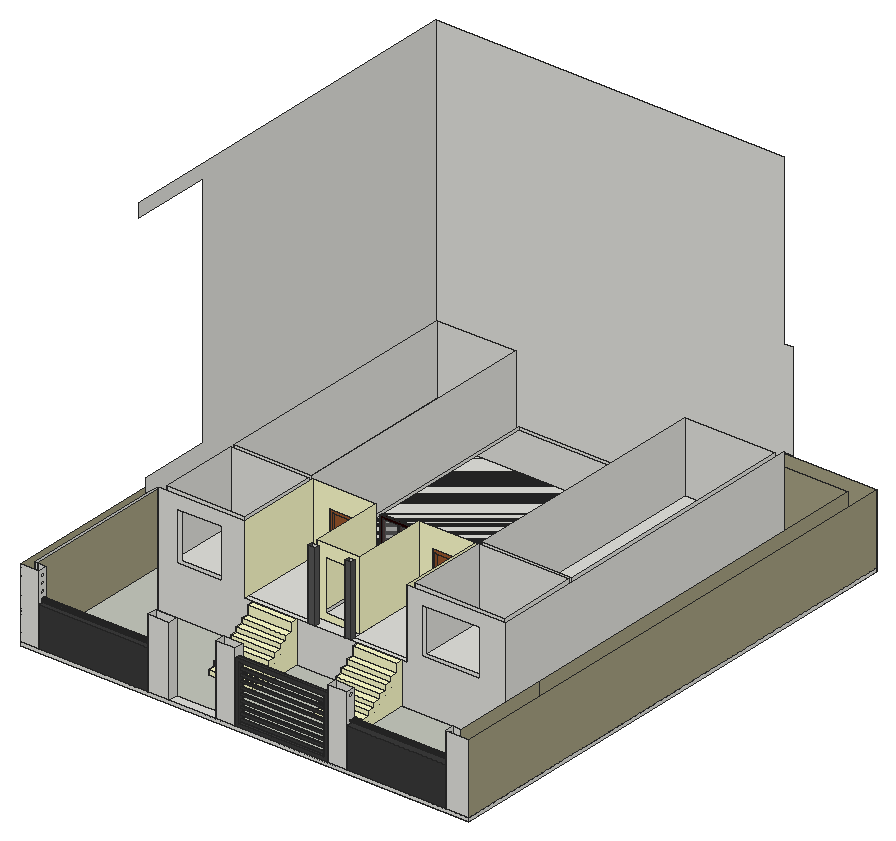
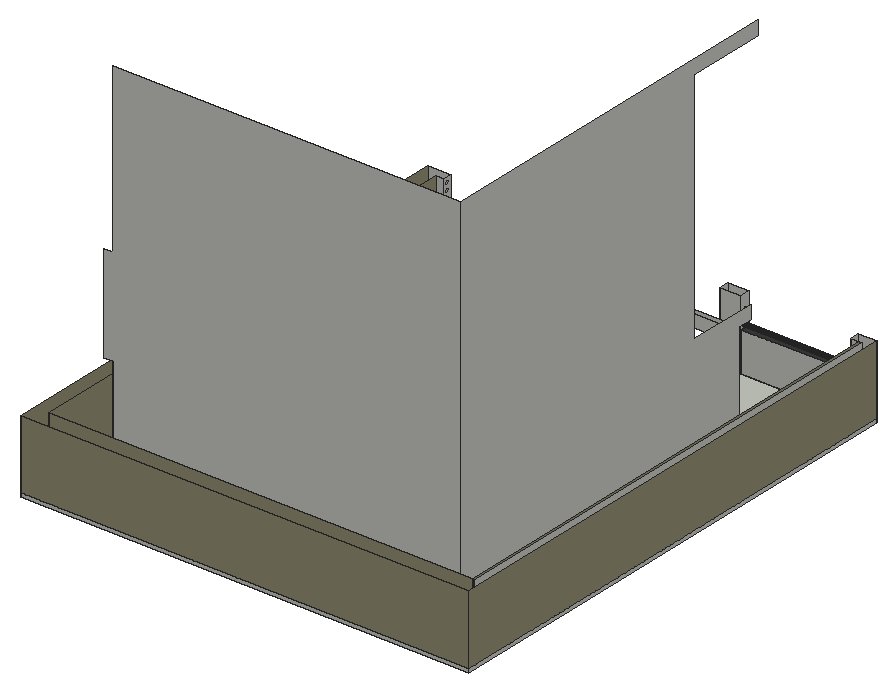
# SketchUp Ruby script. Lengths in inches.
U = 1.inch
M = Sketchup.active_model
def pt(a) = Geom::Point3d.new(a.map { |v| v * U })
def face(e, loops, mat)
  f = e.add_face(loops[0].map { |a| pt(a) })
  loops[1..].each { |l| e.add_face(l.map { |a| pt(a) }).erase! }
  f.material = f.back_material = mat if mat
  f
end
# faces: each face lists its corners as indices into pts; further lists are holes
def faces(e, pts, list, mat = nil) = list.each { |f| face(e, (f[0].is_a?(Array) ? f : [f]).map { |l| l.map { |i| pts[i] } }, mat) }
# xy, xz, yz: faces in a plane at the given z, y or x. An outline is a flat list of corners, or four numbers for a rectangle; further outlines are holes
def ring(l) = l.size == 4 ? [[l[0], l[1]], [l[2], l[1]], [l[2], l[3]], [l[0], l[3]]] : l.each_slice(2).to_a
def flat(e, list, mat, &to3) = list.each { |f| face(e, (f[0].is_a?(Array) ? f : [f]).map { |l| ring(l).map { |u, v| to3.(u, v) } }, mat) }
def xy(e, z, list, mat = nil) = flat(e, list, mat) { |x, y| [x, y, z] }
def xz(e, y, list, mat = nil) = flat(e, list, mat) { |x, z| [x, y, z] }
def yz(e, x, list, mat = nil) = flat(e, list, mat) { |y, z| [x, y, z] }
def lines(e, pts, list) = list.each { |a, b| e.add_line(pt(pts[a]), pt(pts[b])) }
# prism: a flat outline (further loops are holes) pulled along v
def prism(e, loops, v, mat = nil)
  f = face(e, loops, mat); d = Geom::Vector3d.new(v.map { |x| x * U })
  f.pushpull(f.normal.samedirection?(d) ? d.length : -d.length)
end
def box(e, o, s, mat = nil) = prism(e, [[o, [o[0] + s[0], o[1], o[2]], [o[0] + s[0], o[1] + s[1], o[2]], [o[0], o[1] + s[1], o[2]]]], [0, 0, s[2]], mat)
def at(x, y, z, deg = 0) = Geom::Transformation.translation(pt([x, y, z])) * Geom::Transformation.rotation(ORIGIN, Z_AXIS, deg.degrees)
def axes(o, x, y, z) = Geom::Transformation.new([*x, 0, *y, 0, *z, 0, *pt(o).to_a, 1])
def part(name) = M.definitions.add(name)
# library, detail: a bought-in or finely detailed component or shape, given as its bounding box
def library(name, o, s) = part(name).tap { |d| box(d.entities, o, s) }
def detail(e, o, s) = box(e.add_group.entities, o, s)
def put(e, d, t, mat = nil) = e.add_instance(d, t).tap { |i| i.material = mat if mat }
def group(e, t, mat = nil) = e.add_group.tap { |g| g.transformation = t; g.material = mat if mat }.entities
root = M.entities
M.materials.add("[Color A08]").color = [30, 0, 0]
M.materials.add("[Color E01]").color = [255, 255, 204]
M.materials.add("[Color M06]").color = [86, 86, 86]
M.materials.add("[Color M07]").color = [58, 58, 58]
M.materials.add("[Pavers with Grass Herringbone]").color = [197, 201, 190]
M.materials.add("[Stone Coursed Rough]").color = [165, 160, 130]
M.materials.add("[Translucent Glass Gray]").color = [128, 128, 128]
M.materials["[Translucent Glass Gray]"].alpha = 0.5
M.materials.add("[Wood Cherry Original]").color = [152, 86, 42]
c1 = part("Group\#3")
xy(c1.entities,0,[[0,0,60.375,4]])
xy(c1.entities,4.67,[[4.67,0,28.45,4],[32.75,0,55.71,4]],"[Color A08]")
xy(c1.entities,93.02,[[4.67,0,28.45,4],[32.75,0,55.71,4]])
xy(c1.entities,97.6875,[[0,0,60.375,4]],"[Color A08]")
xz(c1.entities,0,[[[0,0,60.375,97.6875],[4.67,4.67,28.45,93.02],[32.75,4.67,55.71,93.02]]],"[Color A08]")
xz(c1.entities,0,[[4.67,4.67,28.45,93.02],[32.75,4.67,55.71,93.02]],"[Translucent Glass Gray]")
xz(c1.entities,4,[[[0,0,60.375,97.6875],[4.67,4.67,28.45,93.02],[32.75,4.67,55.71,93.02]]],"[Color A08]")
yz(c1.entities,0,[[0,0,4,97.6875]],"[Color A08]")
yz(c1.entities,4.67,[[0,4.67,4,93.02]],"[Color A08]")
yz(c1.entities,28.45,[[0,4.67,4,93.02]],"[Color A08]")
yz(c1.entities,32.75,[[0,4.67,4,93.02]],"[Color A08]")
yz(c1.entities,55.71,[[0,4.67,4,93.02]],"[Color A08]")
yz(c1.entities,60.375,[[0,0,4,97.6875]],"[Color A08]")
c2 = part("Group\#1")
xy(c2.entities,0,[[0,0,48,9.0625]],"[Wood Cherry Original]")
xy(c2.entities,4.61,[[4.61,0,43.39,3.0625],[4.61,3.0625,43.39,9.0625]],"[Wood Cherry Original]")
xy(c2.entities,79.39,[[4.61,0,43.39,3.0625],[4.61,3.0625,43.39,9.0625]],"[Wood Cherry Original]")
xy(c2.entities,84,[[0,0,48,9.0625]],"[Wood Cherry Original]")
xz(c2.entities,0,[[[0,0,48,84],[4.61,4.61,43.39,79.39]]],"[Wood Cherry Original]")
xz(c2.entities,3.0625,[[4.61,4.61,43.39,79.39]],"[Wood Cherry Original]")
xz(c2.entities,9.0625,[[[0,0,48,84],[4.61,4.61,43.39,79.39]]],"[Wood Cherry Original]")
yz(c2.entities,0,[[0,0,9.0625,84]],"[Wood Cherry Original]")
yz(c2.entities,4.61,[[0,4.61,3.0625,79.39],[3.0625,4.61,9.0625,79.39]],"[Wood Cherry Original]")
yz(c2.entities,43.39,[[0,4.61,3.0625,79.39],[3.0625,4.61,9.0625,79.39]],"[Wood Cherry Original]")
yz(c2.entities,48,[[0,0,9.0625,84]],"[Wood Cherry Original]")
xy(root,0,[[0,0,772,183.0625],[0,183.0625,772,878.5]])
xy(root,6,[[0,0,0,878.5,746.625,878.5,746.625,849.54,11.8,849.54,11.8,16.17,31.52,16.17,31.52,0],[31.52,0,219.71,16.17],[219.71,0,256.64,16.17],[256.64,0,336.85,16.17],[336.85,0,370.02,16.17],
  [370.02,0,529.83,16.17],[529.83,0,562.05,16.17],[562.05,0,732.77,16.17],[732.77,0,732.77,16.17,746.625,16.17,746.625,183.0625,772,183.0625,772,0],[11.8,16.17,16.36,849.54],
  [[254.35,87.0625,330.35,87.0625,330.35,183.0625,435.23,183.0625,435.23,87.0625,511.23,87.0625,511.23,183.0625,689.625,183.0625,689.625,783.0625,89.625,783.0625,89.625,183.0625,254.35,183.0625],[746.625,183.0625,772,849.54]],[254.35,87.0625,330.35,99.0625],[435.23,87.0625,511.23,99.0625],[254.35,99.0625,330.35,183.0625],[435.23,99.0625,511.23,183.0625],
  [89.625,183.0625,689.625,783.0625],[746.625,849.54,772,878.5]])
xy(root,6,[[16.36,16.17,746.625,849.54]],"[Pavers with Grass Herringbone]")
xy(root,14,[[254.35,87.0625,330.35,99.0625],[435.23,87.0625,511.23,99.0625]],"[Color E01]")
xy(root,22,[[254.35,99.0625,330.35,111.0625],[435.23,99.0625,511.23,111.0625]],"[Color E01]")
xy(root,30,[[254.35,111.0625,330.35,123.0625],[435.23,111.0625,511.23,123.0625]],"[Color E01]")
xy(root,38,[[254.35,123.0625,330.35,135.0625],[435.23,123.0625,511.23,135.0625]],"[Color E01]")
xy(root,46,[[254.35,135.0625,330.35,147.0625],[435.23,135.0625,511.23,147.0625]],"[Color E01]")
xy(root,54,[[254.35,147.0625,330.35,159.0625],[435.23,147.0625,511.23,159.0625]],"[Color E01]")
xy(root,62,[[254.35,159.0625,330.35,171.0625],[435.23,159.0625,511.23,171.0625]],"[Color E01]")
xy(root,74.0625,[[31.52,0,219.71,16.17],[562.05,0,732.77,16.17]],"[Color M07]")
xy(root,76.875,[[239.625,183.0625,348.1875,192.0625],[348.1875,183.0625,360.82,192.0625],[360.82,183.0625,360.82,192.0625,348.1875,192.0625,348.1875,203.5,422.35,203.5,422.35,192.0625,412.84,192.0625,412.84,183.0625],[412.84,183.0625,422.35,192.0625],[422.35,183.0625,519.875,192.0625],
  [98.625,192.0625,233.625,330.0625],[239.625,192.0625,348.1875,192.0625,348.1875,330.0625,317.59,330.0625,317.59,336.0625,269.59,336.0625,269.59,330.0625,239.625,330.0625],[422.35,192.0625,519.875,192.0625,519.875,330.0625,494.24,330.0625,494.24,336.0625,446.24,336.0625,446.24,330.0625,422.35,330.0625],[525.875,192.0625,680.625,330.0625],[348.1875,203.5,348.1875,330.0625,317.59,330.0625,317.59,336.0625,351.23,336.0625,351.23,209.5625,418.5,209.5625,418.5,336.0625,446.24,336.0625,446.24,330.0625,422.35,330.0625,422.35,203.5],
  [98.625,336.0625,233.625,774.0625],[525.875,336.0625,680.625,774.0625]])
xy(root,76.875,[[254.35,171.0625,330.35,183.0625],[435.23,171.0625,511.23,183.0625]],"[Color E01]")
xz(root,0,[[0,0,772,6],[0,6,31.52,126],[219.71,6,256.64,126],[336.85,6,370.02,126],[529.83,6,562.05,126],
  [732.77,6,772,126]])
xz(root,0,[[31.52,6,219.71,74.0625],[562.05,6,732.77,74.0625]],"[Color M07]")
xz(root,16.17,[[11.8,6,16.36,126],[16.36,6,31.52,126],[31.52,6,219.71,74.0625],[219.71,6,256.64,126],[336.85,6,370.02,126],
  [529.83,6,562.05,126],[562.05,6,732.77,74.0625],[732.77,6,746.625,126]])
xz(root,87.0625,[[254.35,6,330.35,14],[435.23,6,511.23,14]],"[Color E01]")
xz(root,99.0625,[[254.35,14,330.35,22],[435.23,14,511.23,22]],"[Color E01]")
xz(root,111.0625,[[254.35,22,330.35,30],[435.23,22,511.23,30]],"[Color E01]")
xz(root,123.0625,[[254.35,30,330.35,38],[435.23,30,511.23,38]],"[Color E01]")
xz(root,135.0625,[[254.35,38,330.35,46],[435.23,38,511.23,46]],"[Color E01]")
xz(root,147.0625,[[254.35,46,330.35,54],[435.23,46,511.23,54]],"[Color E01]")
xz(root,159.0625,[[254.35,54,330.35,62],[435.23,54,511.23,62]],"[Color E01]")
xz(root,171.0625,[[254.35,62,330.35,76.875],[435.23,62,511.23,76.875]],"[Color E01]")
xz(root,183.0625,[[[89.625,6,254.35,6,254.35,76.875,239.625,76.875,239.625,196.875,89.625,196.875],[124.03,90.39,201.03,175.07]],[254.35,6,330.35,76.875],[330.35,6,435.23,76.875],[435.23,6,511.23,76.875],[[511.23,6,689.625,6,689.625,196.875,519.875,196.875,519.875,76.875,511.23,76.875],[545.68,95.4,644.56,174.78]]])
xz(root,183.0625,[[348.1875,76.875,360.82,196.875],[412.84,76.875,422.35,196.875]],"[Color M06]")
xz(root,192.0625,[[[98.625,76.875,233.625,196.875],[124.03,90.39,201.03,175.07]],[348.1875,76.875,360.82,196.875],[412.84,76.875,422.35,196.875],[[525.875,76.875,680.625,196.875],[545.68,95.4,644.56,174.78]]])
xz(root,203.5,[[[348.1875,76.875,422.35,196.875],[362.91,88.1,408.97,174.47]]],"[Color E01]")
xz(root,209.5625,[[351.23,76.875,418.5,81.5625]])
xz(root,330.0625,[[98.625,76.875,233.625,196.875],[525.875,76.875,680.625,196.875]])
xz(root,330.0625,[[239.625,76.875,269.59,76.875,269.59,160.875,317.59,160.875,317.59,76.875,348.1875,76.875,348.1875,196.875,239.625,196.875],[422.35,76.875,446.24,76.875,446.24,160.875,494.24,160.875,494.24,76.875,519.875,76.875,519.875,196.875,422.35,196.875]],"[Color E01]")
xz(root,336.0625,[[98.625,76.875,233.625,196.875],[239.625,76.875,269.59,81.5625],[269.59,76.875,317.59,81.5625],[317.59,76.875,351.23,81.5625],[418.5,76.875,446.24,81.5625],
  [494.24,76.875,519.875,81.5625],[525.875,76.875,680.625,196.875]])
xz(root,774.0625,[[98.625,76.875,233.625,196.875],[239.625,76.875,519.875,81.5625],[525.875,76.875,680.625,196.875]])
xz(root,783.0625,[[89.625,6,89.625,652.875,689.625,652.875,689.625,364.875,704.125,364.875,704.125,196.875,689.625,196.875,689.625,6]])
xz(root,849.54,[[11.8,6,16.36,126]])
xz(root,849.54,[[16.36,6,746.625,126]],"[Stone Coursed Rough]")
xz(root,878.5,[[0,0,772,6]])
xz(root,878.5,[[0,6,772,126]],"[Stone Coursed Rough]")
yz(root,0,[[0,0,878.5,6]])
yz(root,0,[[0,6,878.5,126]],"[Stone Coursed Rough]")
yz(root,11.8,[[16.17,6,849.54,126]])
yz(root,16.36,[[16.17,6,849.54,126]],"[Stone Coursed Rough]")
yz(root,31.52,[[0,6,16.17,74.0625],[[0,74.0625,16.17,126],[8.45,101.5,7.61,101.61,6.83,101.93,6.15,102.45,5.64,103.12,5.3125,103.91,5.2,104.75,5.3125,105.59,5.64,106.37,6.15,107.05,6.83,107.5625,7.61,107.89,8.45,108,9.29,107.89,10.08,107.5625,10.75,107.05,11.27,106.37,11.59,105.59,11.7,104.75,11.59,103.91,11.27,103.12,10.75,102.45,10.08,101.93,9.29,101.61],[8.45,88,7.61,88.11,6.83,88.43,6.15,88.95,5.64,89.62,5.3125,90.41,5.2,91.25,5.3125,92.09,5.64,92.87,6.15,93.55,6.83,94.0625,7.61,94.39,8.45,94.5,9.29,94.39,10.08,94.0625,10.75,93.55,11.27,92.87,11.59,92.09,11.7,91.25,11.59,90.41,11.27,89.62,10.75,88.95,10.08,88.43,9.29,88.11],[8.45,76,7.61,76.11,6.83,76.43,6.15,76.95,5.64,77.62,5.3125,78.41,5.2,79.25,5.3125,80.09,5.64,80.87,6.15,81.55,6.83,82.0625,7.61,82.39,8.45,82.5,9.29,82.39,10.08,82.0625,10.75,81.55,11.27,80.87,11.59,80.09,11.7,79.25,11.59,78.41,11.27,77.62,10.75,76.95,10.08,76.43,9.29,76.11],[8.45,113.18,7.61,113.3,6.83,113.62,6.15,114.14,5.64,114.81,5.3125,115.59,5.2,116.43,5.3125,117.28,5.64,118.06,6.15,118.73,6.83,119.25,7.61,119.57,8.45,119.68,9.29,119.57,10.08,119.25,10.75,118.73,11.27,118.06,11.59,117.28,11.7,116.43,11.59,115.59,11.27,114.81,10.75,114.14,10.08,113.62,9.29,113.3]]])
yz(root,89.625,[[183.0625,6,183.0625,196.875,159.1875,196.875,159.1875,220.875,281.125,220.875,281.125,628.875,142.25,628.875,142.25,652.875,783.0625,652.875,783.0625,6]])
yz(root,98.625,[[192.0625,76.875,330.0625,196.875],[336.0625,76.875,774.0625,196.875]])
yz(root,219.71,[[0,6,16.17,74.0625],[[0,74.0625,16.17,126],[8.45,101.5,9.29,101.61,10.08,101.93,10.75,102.45,11.27,103.12,11.59,103.91,11.7,104.75,11.59,105.59,11.27,106.37,10.75,107.05,10.08,107.5625,9.29,107.89,8.45,108,7.61,107.89,6.83,107.5625,6.15,107.05,5.64,106.37,5.3125,105.59,5.2,104.75,5.3125,103.91,5.64,103.12,6.15,102.45,6.83,101.93,7.61,101.61]]])
yz(root,221.4,[[8.45,76,9.29,76.11,10.08,76.43,10.75,76.95,11.27,77.62,11.59,78.41,11.7,79.25,11.59,80.09,11.27,80.87,10.75,81.55,10.08,82.0625,9.29,82.39,8.45,82.5,7.61,82.39,6.83,82.0625,6.15,81.55,5.64,80.87,5.3125,80.09,5.2,79.25,5.3125,78.41,5.64,77.62,6.15,76.95,6.83,76.43,7.61,76.11]])
yz(root,233.625,[[192.0625,76.875,330.0625,196.875],[336.0625,76.875,774.0625,196.875]])
yz(root,239.625,[[336.0625,76.875,774.0625,81.5625]])
yz(root,239.625,[[183.0625,76.875,330.0625,196.875]],"[Color E01]")
yz(root,254.35,[[87.0625,6,99.0625,14],[99.0625,6,99.0625,22,111.0625,22,111.0625,30,123.0625,30,123.0625,38,135.0625,38,135.0625,46,147.0625,46,147.0625,54,159.0625,54,159.0625,62,171.0625,62,171.0625,76.875,183.0625,76.875,183.0625,6]],"[Color E01]")
yz(root,256.64,[[0,6,16.17,126]])
yz(root,269.59,[[330.0625,76.875,336.0625,160.875]])
yz(root,317.59,[[330.0625,76.875,336.0625,160.875]])
yz(root,330.35,[[87.0625,6,183.0625,6,183.0625,76.875,171.0625,76.875,171.0625,62,159.0625,62,159.0625,54,147.0625,54,147.0625,46,135.0625,46,135.0625,38,123.0625,38,123.0625,30,111.0625,30,111.0625,22,99.0625,22,99.0625,14,87.0625,14]],"[Color E01]")
yz(root,336.85,[[0,6,16.17,126]])
yz(root,348.1875,[[203.5,76.875,330.0625,196.875]],"[Color E01]")
yz(root,348.1875,[[183.0625,76.875,192.0625,196.875]],"[Color M06]")
yz(root,351.23,[[209.5625,76.875,336.0625,81.5625]])
yz(root,360.82,[[183.0625,76.875,192.0625,196.875]],"[Color M06]")
yz(root,370.02,[[0,6,16.17,126]])
yz(root,412.84,[[183.0625,76.875,192.0625,196.875]],"[Color M06]")
yz(root,418.5,[[209.5625,76.875,336.0625,81.5625]])
yz(root,422.35,[[203.5,76.875,330.0625,196.875]],"[Color E01]")
yz(root,422.35,[[183.0625,76.875,192.0625,196.875]],"[Color M06]")
yz(root,435.23,[[171.0625,62,183.0625,76.875]])
yz(root,435.23,[[87.0625,6,87.0625,14,99.0625,14,99.0625,22,111.0625,22,111.0625,30,123.0625,30,123.0625,38,135.0625,38,135.0625,46,147.0625,46,147.0625,54,159.0625,54,159.0625,62,183.0625,62,183.0625,6]],"[Color E01]")
yz(root,446.24,[[330.0625,76.875,336.0625,160.875]])
yz(root,494.24,[[330.0625,76.875,336.0625,160.875]])
yz(root,511.23,[[87.0625,6,183.0625,6,183.0625,76.875,171.0625,76.875,171.0625,62,159.0625,62,159.0625,54,147.0625,54,147.0625,46,135.0625,46,135.0625,38,123.0625,38,123.0625,30,111.0625,30,111.0625,22,99.0625,22,99.0625,14,87.0625,14]],"[Color E01]")
yz(root,519.875,[[336.0625,76.875,774.0625,81.5625]])
yz(root,519.875,[[183.0625,76.875,330.0625,196.875]],"[Color E01]")
yz(root,525.875,[[192.0625,76.875,330.0625,196.875],[336.0625,76.875,774.0625,196.875]])
yz(root,529.83,[[0,6,16.17,126]])
yz(root,561.7,[[8.57,77.6,7.61,77.83,6.73,78.3,6.01,78.99,5.48,79.83,5.2,80.79,5.17,81.78,5.4,82.75,5.875,83.625,6.56,84.35,7.4,84.87,8.36,85.16,9.35,85.1875,10.32,84.96,11.2,84.48,11.92,83.8,12.44,82.95,12.73,82,12.76,81,12.53,80.04,12.05,79.16,11.37,78.4375,10.52,77.91,9.57,77.63]])
yz(root,562.05,[[0,6,16.17,74.0625],[[0,74.0625,16.17,126],[8.57,114.16,7.61,114.39,6.73,114.87,6.01,115.55,5.48,116.4,5.2,117.35,5.17,118.34,5.4,119.3125,5.875,120.1875,6.56,120.91,7.4,121.43,8.36,121.72,9.35,121.75,10.32,121.52,11.2,121.05,11.92,120.36,12.44,119.52,12.73,118.5625,12.76,117.57,12.53,116.6,12.05,115.72,11.37,115,10.52,114.48,9.57,114.19]]])
yz(root,680.625,[[192.0625,76.875,330.0625,196.875],[336.0625,76.875,774.0625,196.875]])
yz(root,689.625,[[183.0625,6,783.0625,196.875]])
yz(root,732.77,[[0,6,16.17,74.0625],[[0,74.0625,16.17,126],[8.57,101.66,9.57,101.69,10.52,101.98,11.37,102.5,12.05,103.22,12.53,104.1,12.76,105.07,12.73,106.0625,12.44,107.02,11.92,107.86,11.2,108.55,10.32,109.02,9.35,109.25,8.36,109.22,7.4,108.93,6.56,108.41,5.875,107.6875,5.4,106.8125,5.17,105.84,5.2,104.85,5.48,103.9,6.01,103.05,6.73,102.37,7.61,101.89],[8.57,89.23,9.57,89.25,10.52,89.54,11.37,90.0625,12.05,90.79,12.53,91.66,12.76,92.63,12.73,93.625,12.44,94.58,11.92,95.42,11.2,96.11,10.32,96.58,9.35,96.8125,8.36,96.78,7.4,96.5,6.56,95.97,5.875,95.25,5.4,94.375,5.17,93.41,5.2,92.41,5.48,91.46,6.01,90.61,6.73,89.93,7.61,89.46],[8.57,77.6,9.57,77.63,10.52,77.91,11.37,78.4375,12.05,79.16,12.53,80.04,12.76,81,12.73,82,12.44,82.95,11.92,83.8,11.2,84.48,10.32,84.96,9.35,85.1875,8.36,85.16,7.4,84.87,6.56,84.35,5.875,83.625,5.4,82.75,5.17,81.78,5.2,80.79,5.48,79.83,6.01,78.99,6.73,78.3,7.61,77.83],[8.57,114.16,9.57,114.19,10.52,114.48,11.37,115,12.05,115.72,12.53,116.6,12.76,117.57,12.73,118.5625,12.44,119.52,11.92,120.36,11.2,121.05,10.32,121.52,9.35,121.75,8.36,121.72,7.4,121.43,6.56,120.91,5.875,120.1875,5.4,119.3125,5.17,118.34,5.2,117.35,5.48,116.4,6.01,115.55,6.73,114.87,7.61,114.39]]])
yz(root,746.625,[[16.17,6,183.0625,126],[183.0625,6,849.54,126]],"[Stone Coursed Rough]")
yz(root,772,[[0,0,878.5,6]])
yz(root,772,[[0,6,878.5,126]],"[Stone Coursed Rough]")
p = [[31.52,7.61,76.11],[31.52,8.45,76],[221.4,8.45,76],[221.4,7.61,76.11],[31.52,9.29,76.11],[221.4,9.29,76.11],
  [31.52,6.83,76.43],[221.4,6.83,76.43],[31.52,10.08,76.43],[221.4,10.08,76.43],[31.52,6.15,76.95],[221.4,6.15,76.95],
  [31.52,10.75,76.95],[221.4,10.75,76.95],[31.52,5.64,77.62],[221.4,5.64,77.62],[31.52,11.27,77.62],[221.4,11.27,77.62],
  [31.52,5.3125,78.41],[221.4,5.3125,78.41],[732.77,8.57,77.6],[732.77,7.61,77.83],[561.7,7.61,77.83],[561.7,8.57,77.6],
  [732.77,9.57,77.63],[561.7,9.57,77.63],[732.77,10.52,77.91],[561.7,10.52,77.91],[31.52,11.59,78.41],[221.4,11.59,78.41],
  [732.77,6.73,78.3],[561.7,6.73,78.3],[732.77,11.37,78.4375],[561.7,11.37,78.4375],[732.77,6.01,78.99],[561.7,6.01,78.99],
  [31.52,5.2,79.25],[221.4,5.2,79.25],[732.77,12.05,79.16],[561.7,12.05,79.16],[31.52,11.7,79.25],[221.4,11.7,79.25],
  [732.77,5.48,79.83],[561.7,5.48,79.83],[31.52,5.3125,80.09],[221.4,5.3125,80.09],[31.52,11.59,80.09],[221.4,11.59,80.09],
  [732.77,12.53,80.04],[561.7,12.53,80.04],[732.77,5.2,80.79],[561.7,5.2,80.79],[732.77,12.76,81],[561.7,12.76,81],
  [31.52,5.64,80.87],[221.4,5.64,80.87],[31.52,11.27,80.87],[221.4,11.27,80.87],[732.77,5.17,81.78],[561.7,5.17,81.78],
  [31.52,6.15,81.55],[221.4,6.15,81.55],[31.52,10.75,81.55],[221.4,10.75,81.55],[732.77,12.73,82],[561.7,12.73,82],
  [353.67,336.0625,58.9375],[353.67,336.0625,76.875],[330.35,147.0625,38],[254.35,147.0625,38],[330.35,135.0625,30],[254.35,135.0625,30],
  [330.35,123.0625,22],[254.35,123.0625,22],[330.35,111.0625,14],[254.35,111.0625,14],[511.23,159.0625,46],[435.23,159.0625,46],
  [511.23,147.0625,38],[435.23,147.0625,38],[511.23,135.0625,30],[435.23,135.0625,30],[511.23,123.0625,22],[435.23,123.0625,22],
  [511.23,111.0625,14],[435.23,111.0625,14]]
faces(root,p,[[0,1,2,3],[1,4,5,2],[6,0,3,7],[4,8,9,5],[10,6,7,11],[8,12,13,9],[14,10,11,15],[12,16,17,13],
  [18,14,15,19],[20,21,22,23],[24,20,23,25],[26,24,25,27],[16,28,29,17],[21,30,31,22],[32,26,27,33],[30,34,35,31],
  [36,18,19,37],[38,32,33,39],[28,40,41,29],[34,42,43,35],[44,36,37,45],[40,46,47,41],[48,38,39,49],[42,50,51,43],
  [52,48,49,53],[54,44,45,55],[46,56,57,47],[50,58,59,51],[60,54,55,61],[56,62,63,57],[64,52,53,65]],"[Color M07]")
lines(root,p,[[66,67],[68,69],[70,71],[72,73],[74,75],[76,77],[78,79],[80,81],[82,83],[84,85]])
g1 = group(root,at(370.02,0,6))
xy(g1,0,[[0,0,159.8125,6]],"[Color M07]")
xy(g1,5.96,[[6.65,0,153.17,6]],"[Color M07]")
xy(g1,9.68,[[6.65,1.55,155.41,3.55]],"[Color M07]")
xy(g1,13.59,[[6.65,1.55,155.41,3.55]],"[Color M07]")
xy(g1,19.58,[[6.65,1.55,156.25,3.55]],"[Color M07]")
xy(g1,23.5,[[6.65,1.55,156.25,3.55]],"[Color M07]")
xy(g1,29.49,[[6.65,1.55,156,3.55]],"[Color M07]")
xy(g1,33.41,[[6.65,1.55,156,3.55]],"[Color M07]")
xy(g1,39.4,[[6.65,1.55,153.22,3.55]],"[Color M07]")
xy(g1,43.3125,[[6.65,1.55,153.22,3.55]],"[Color M07]")
xy(g1,49.3,[[6.65,1.55,153.17,3.55]],"[Color M07]")
xy(g1,53.22,[[6.65,1.55,153.17,3.55]],"[Color M07]")
xy(g1,59.21,[[6.65,1.55,153.17,3.55]],"[Color M07]")
xy(g1,63.125,[[6.65,1.55,153.17,3.55]],"[Color M07]")
xy(g1,69.12,[[6.65,1.55,153.17,3.55]],"[Color M07]")
xy(g1,73.03,[[6.65,1.55,153.17,3.55]],"[Color M07]")
xy(g1,79.02,[[6.65,1.55,152.71,3.55]],"[Color M07]")
xy(g1,82.94,[[6.65,1.55,152.71,3.55]],"[Color M07]")
xy(g1,88.93,[[6.65,1.55,153.17,3.55]],"[Color M07]")
xy(g1,92.85,[[6.65,1.55,153.17,3.55]],"[Color M07]")
xy(g1,100.75,[[6.65,0,153.17,6]],"[Color M07]")
xy(g1,106.71,[[0,0,159.8125,6]],"[Color M07]")
xz(g1,0,[[[0,0,159.8125,106.71],[6.65,5.96,153.17,100.75]]],"[Color M07]")
xz(g1,1.55,[[6.65,9.68,155.41,13.59],[6.65,19.58,156.25,23.5],[6.65,29.49,156,33.41],[6.65,39.4,153.22,43.3125],[6.65,49.3,153.17,53.22],
  [6.65,59.21,153.17,63.125],[6.65,69.12,153.17,73.03],[6.65,79.02,152.71,82.94],[6.65,88.93,153.17,92.85]],"[Color M07]")
xz(g1,3.55,[[6.65,9.68,155.41,13.59],[6.65,19.58,156.25,23.5],[6.65,29.49,156,33.41],[6.65,39.4,153.22,43.3125],[6.65,49.3,153.17,53.22],
  [6.65,59.21,153.17,63.125],[6.65,69.12,153.17,73.03],[6.65,79.02,152.71,82.94],[6.65,88.93,153.17,92.85]],"[Color M07]")
xz(g1,6,[[[0,0,159.8125,106.71],[6.65,5.96,153.17,100.75]]],"[Color M07]")
yz(g1,0,[[0,0,6,106.71]],"[Color M07]")
yz(g1,6.65,[[1.55,9.68,3.55,13.59],[1.55,19.58,3.55,23.5],[1.55,29.49,3.55,33.41],[1.55,39.4,3.55,43.3125],[1.55,49.3,3.55,53.22],
  [1.55,59.21,3.55,63.125],[1.55,69.12,3.55,73.03],[1.55,79.02,3.55,82.94],[1.55,88.93,3.55,92.85]])
yz(g1,6.65,[[[0,5.96,6,100.75],[1.55,88.93,3.55,92.85],[1.55,79.02,3.55,82.94],[1.55,69.12,3.55,73.03],[1.55,59.21,3.55,63.125],[1.55,49.3,3.55,53.22],[1.55,39.4,3.55,43.3125],[1.55,29.49,3.55,33.41],[1.55,19.58,3.55,23.5],[1.55,9.68,3.55,13.59]]],"[Color M07]")
yz(g1,152.71,[[1.55,79.02,3.55,82.94]])
yz(g1,153.17,[[[0,5.96,6,100.75],[1.55,88.93,3.55,92.85],[1.55,69.12,3.55,73.03],[1.55,49.3,3.55,53.22],[1.55,59.21,3.55,63.125]]],"[Color M07]")
yz(g1,153.22,[[1.55,39.4,3.55,43.3125]])
yz(g1,155.41,[[1.55,9.68,3.55,13.59]])
yz(g1,156,[[1.55,29.49,3.55,33.41]])
yz(g1,156.25,[[1.55,19.58,3.55,23.5]])
yz(g1,159.8125,[[0,0,6,106.71]],"[Color M07]")
put(root,c1,axes([354.2,331.8,76.875],[1.065,0,0],[0,1.065,0],[0,0,1.065]))
put(root,c2,at(269.59,330.0625,76.875))
put(root,c2,at(446.24,330.0625,76.875))
